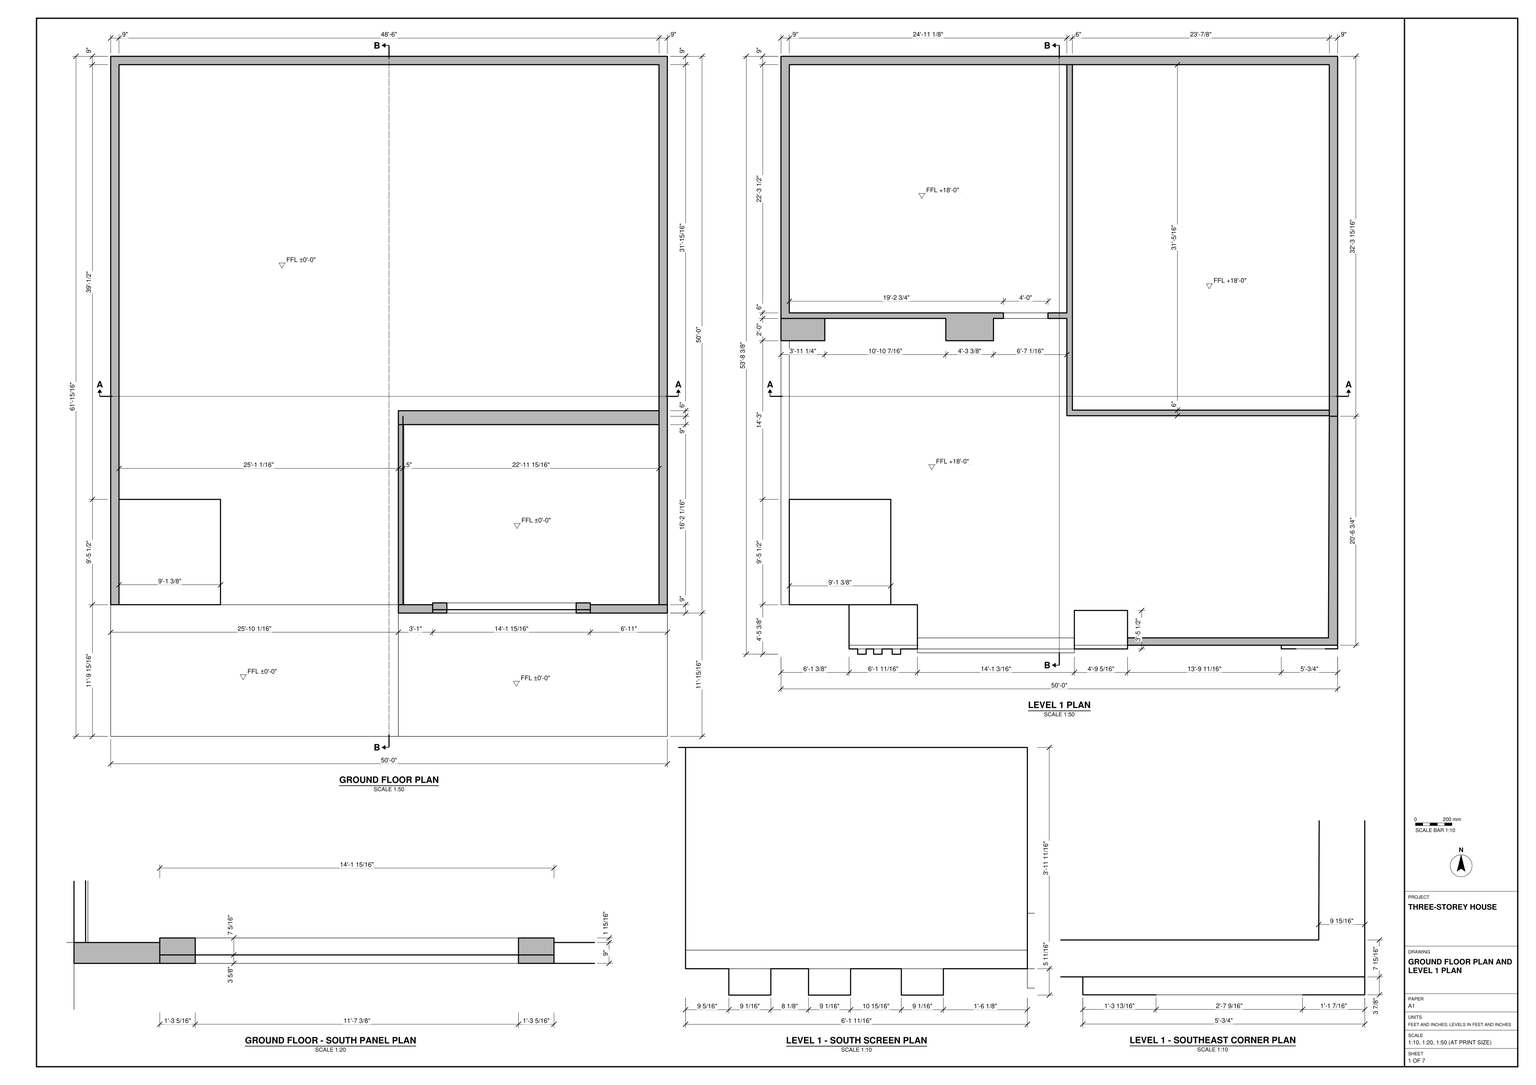
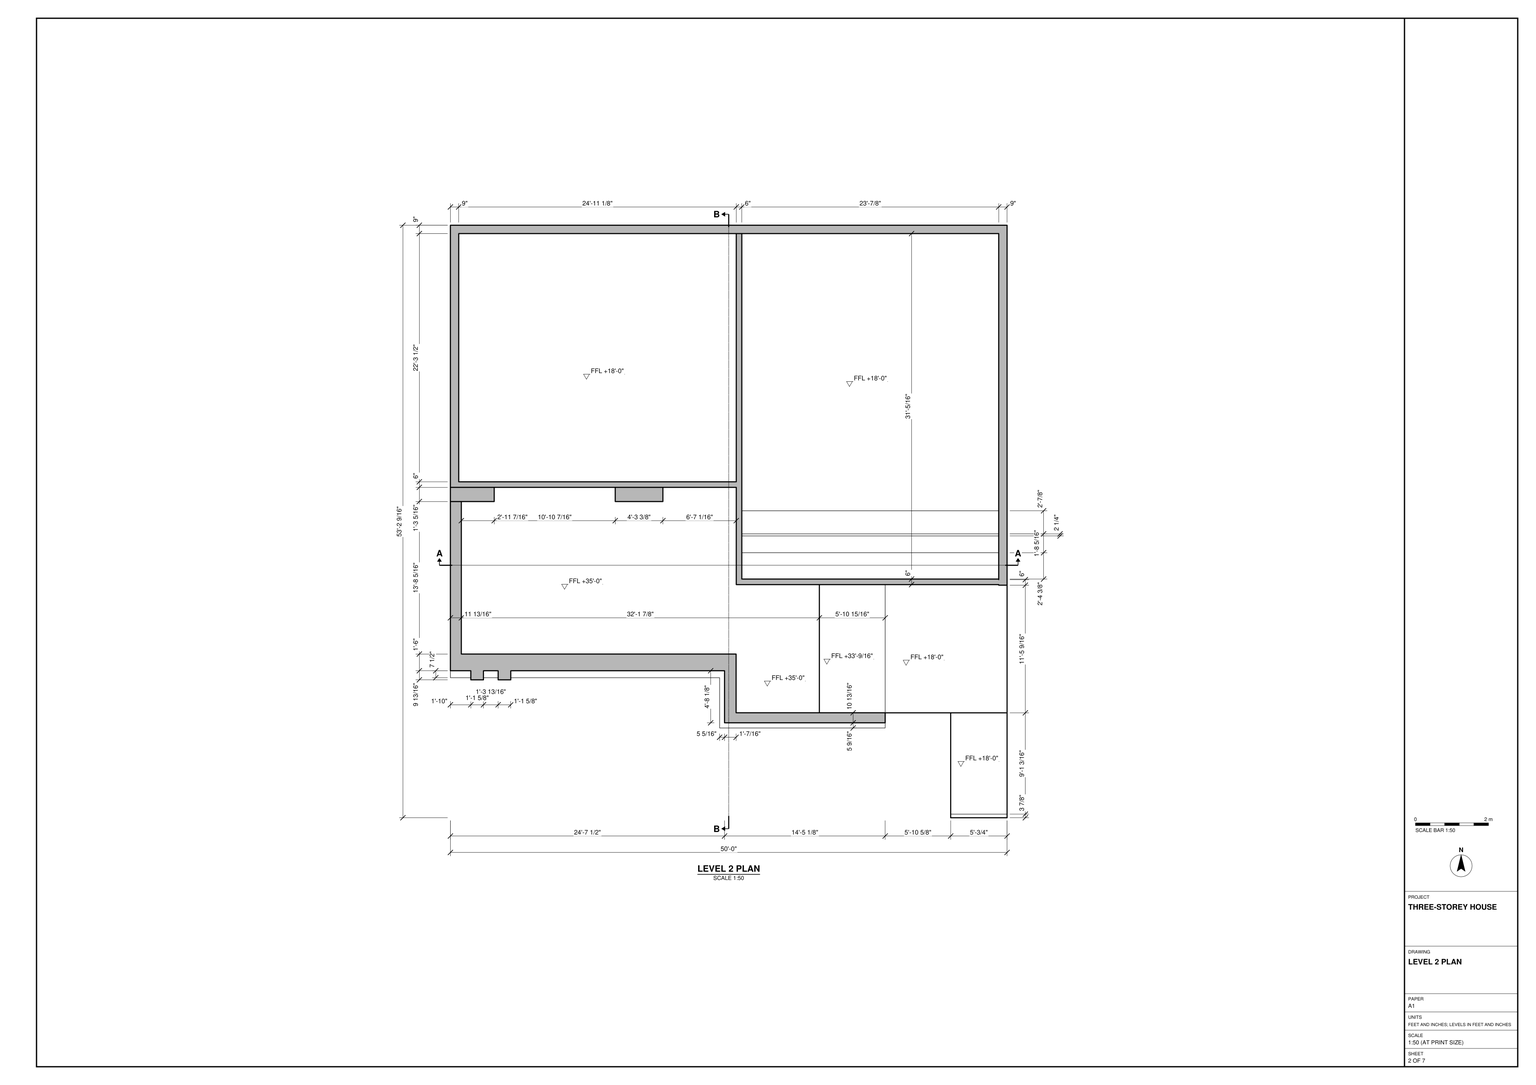
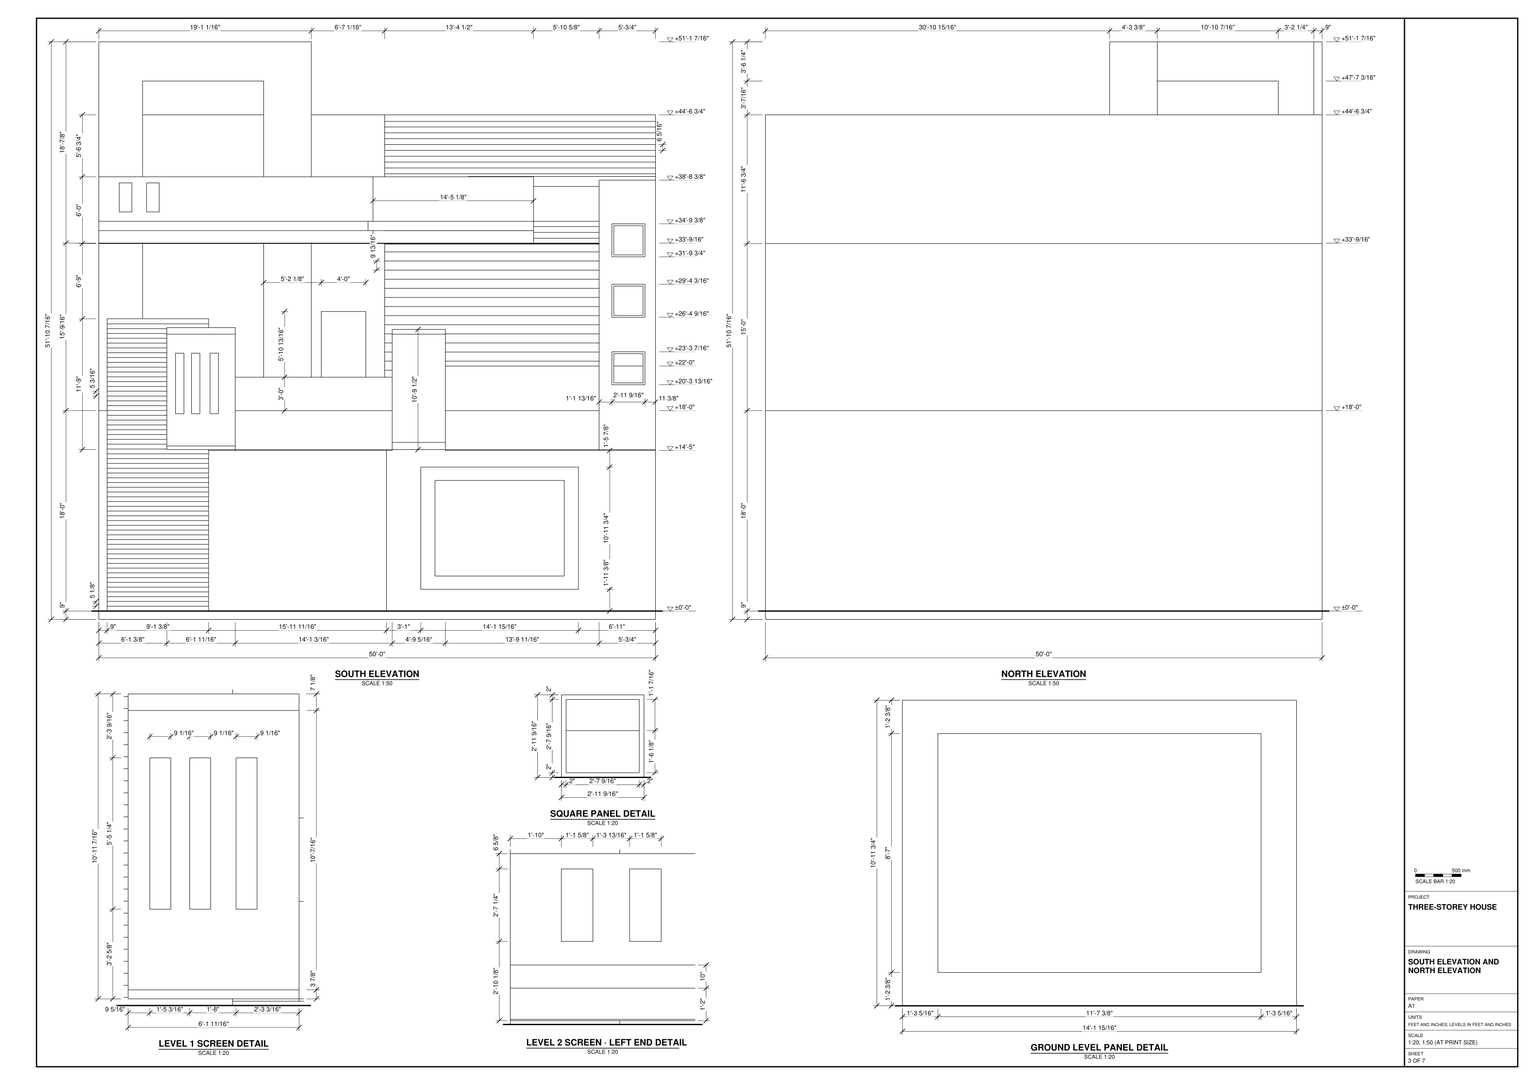
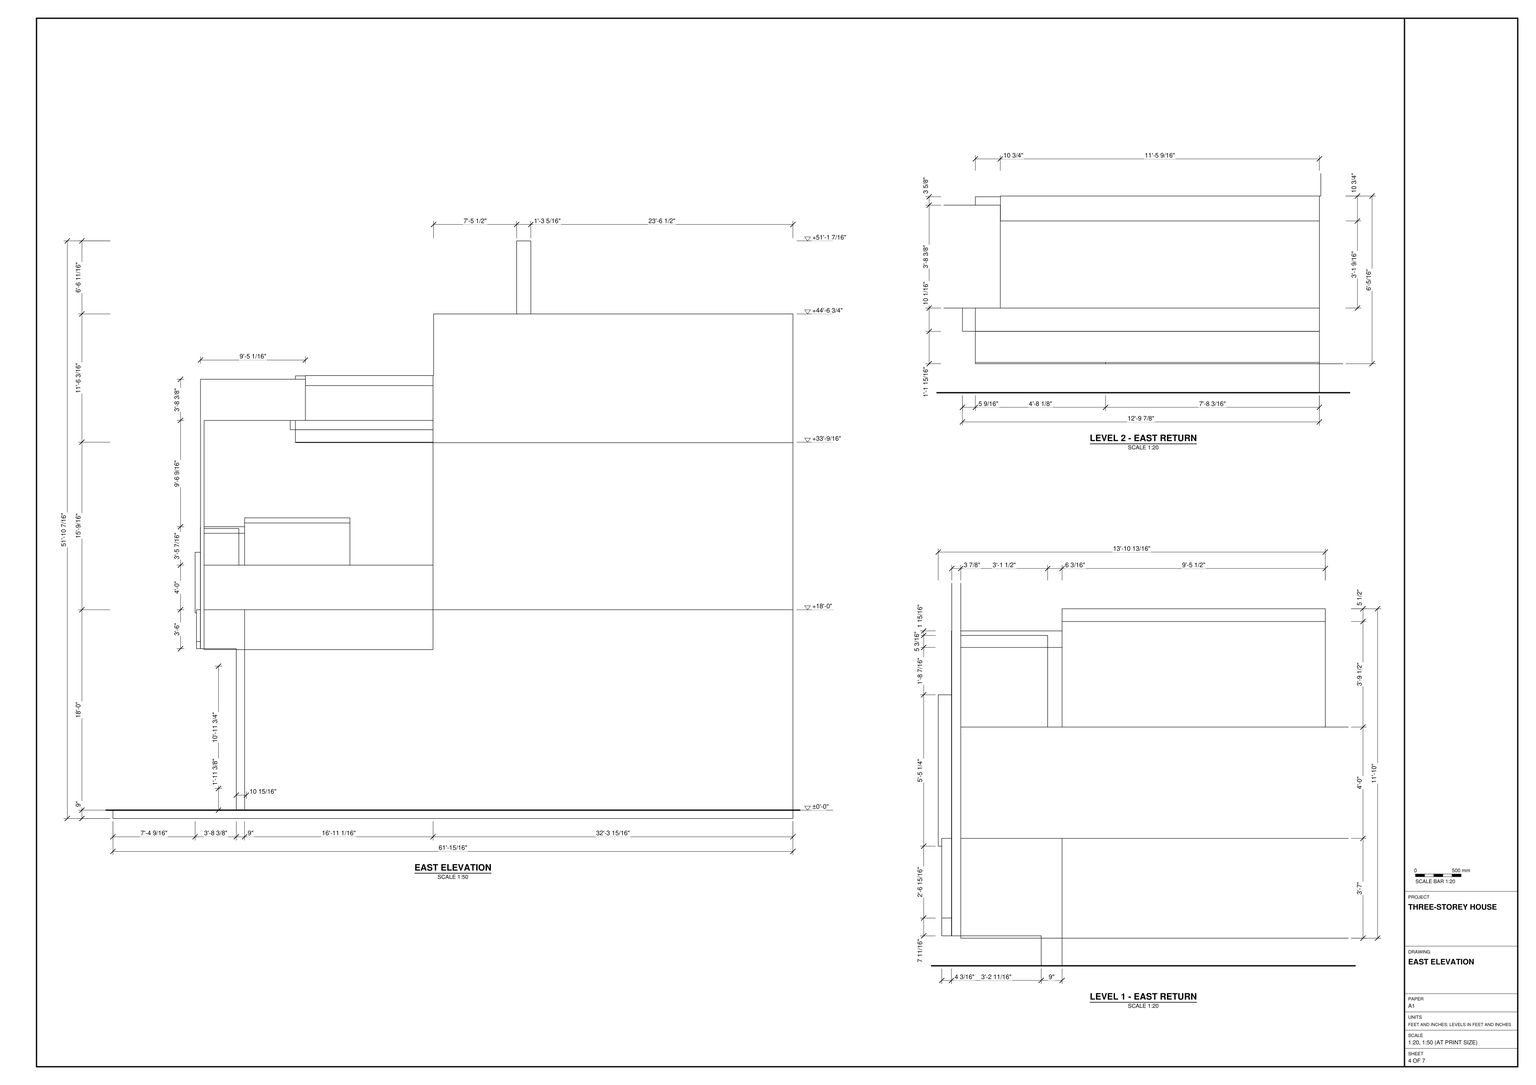
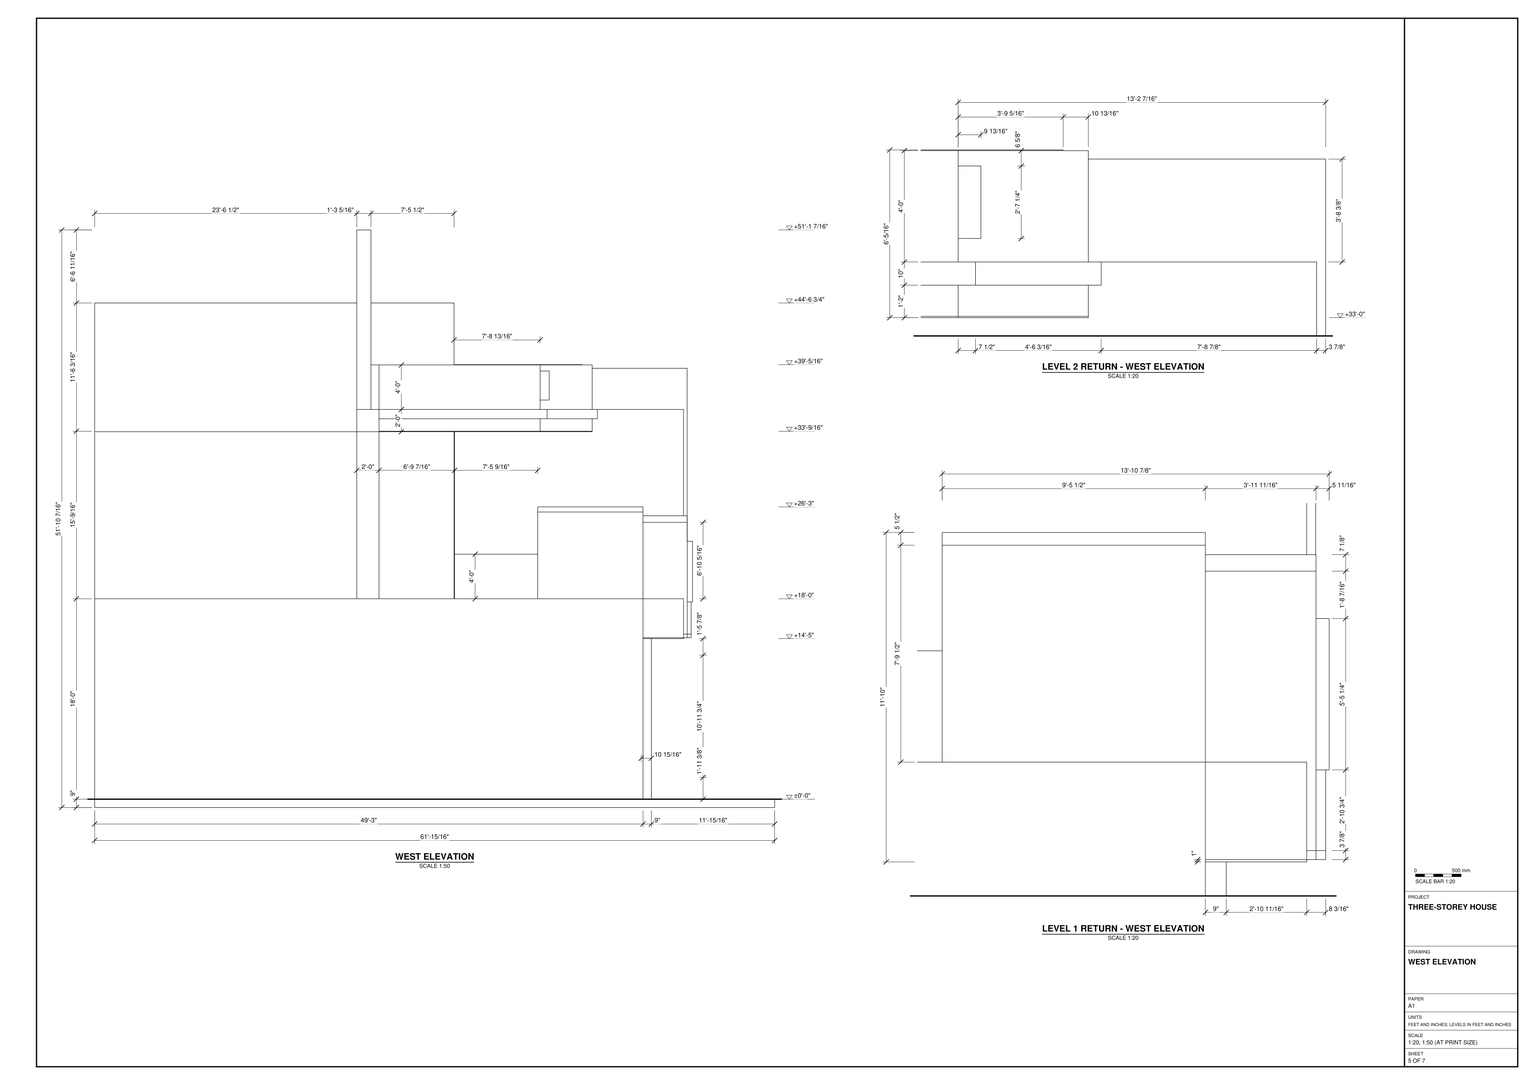
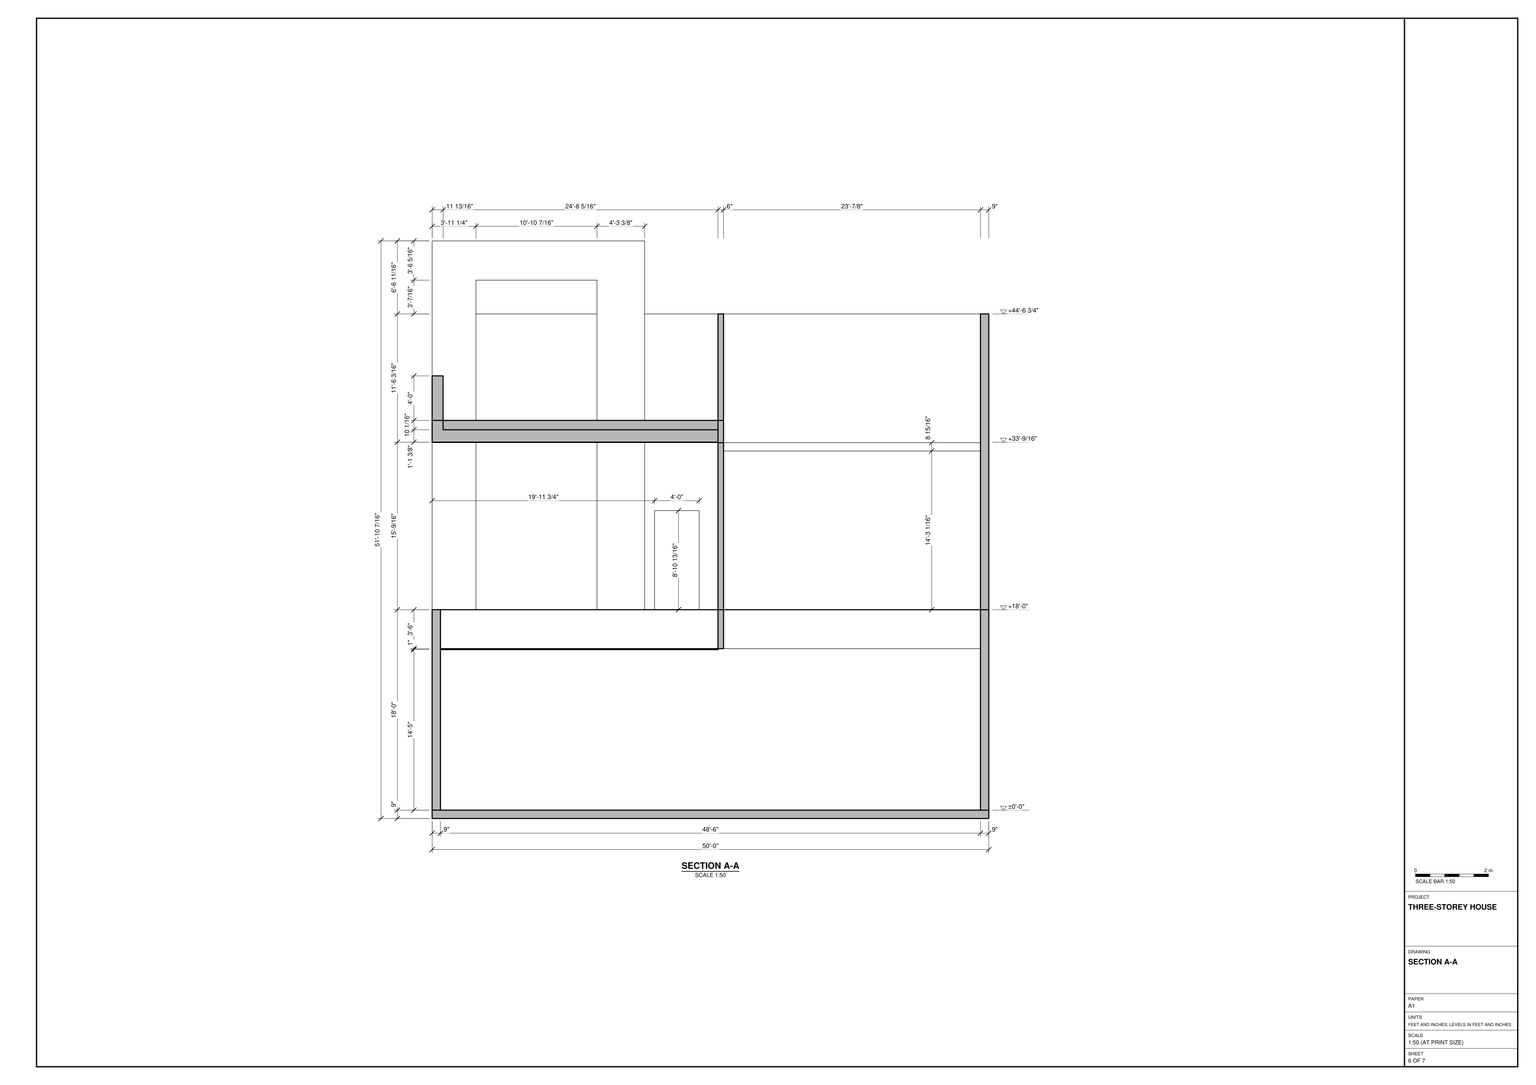
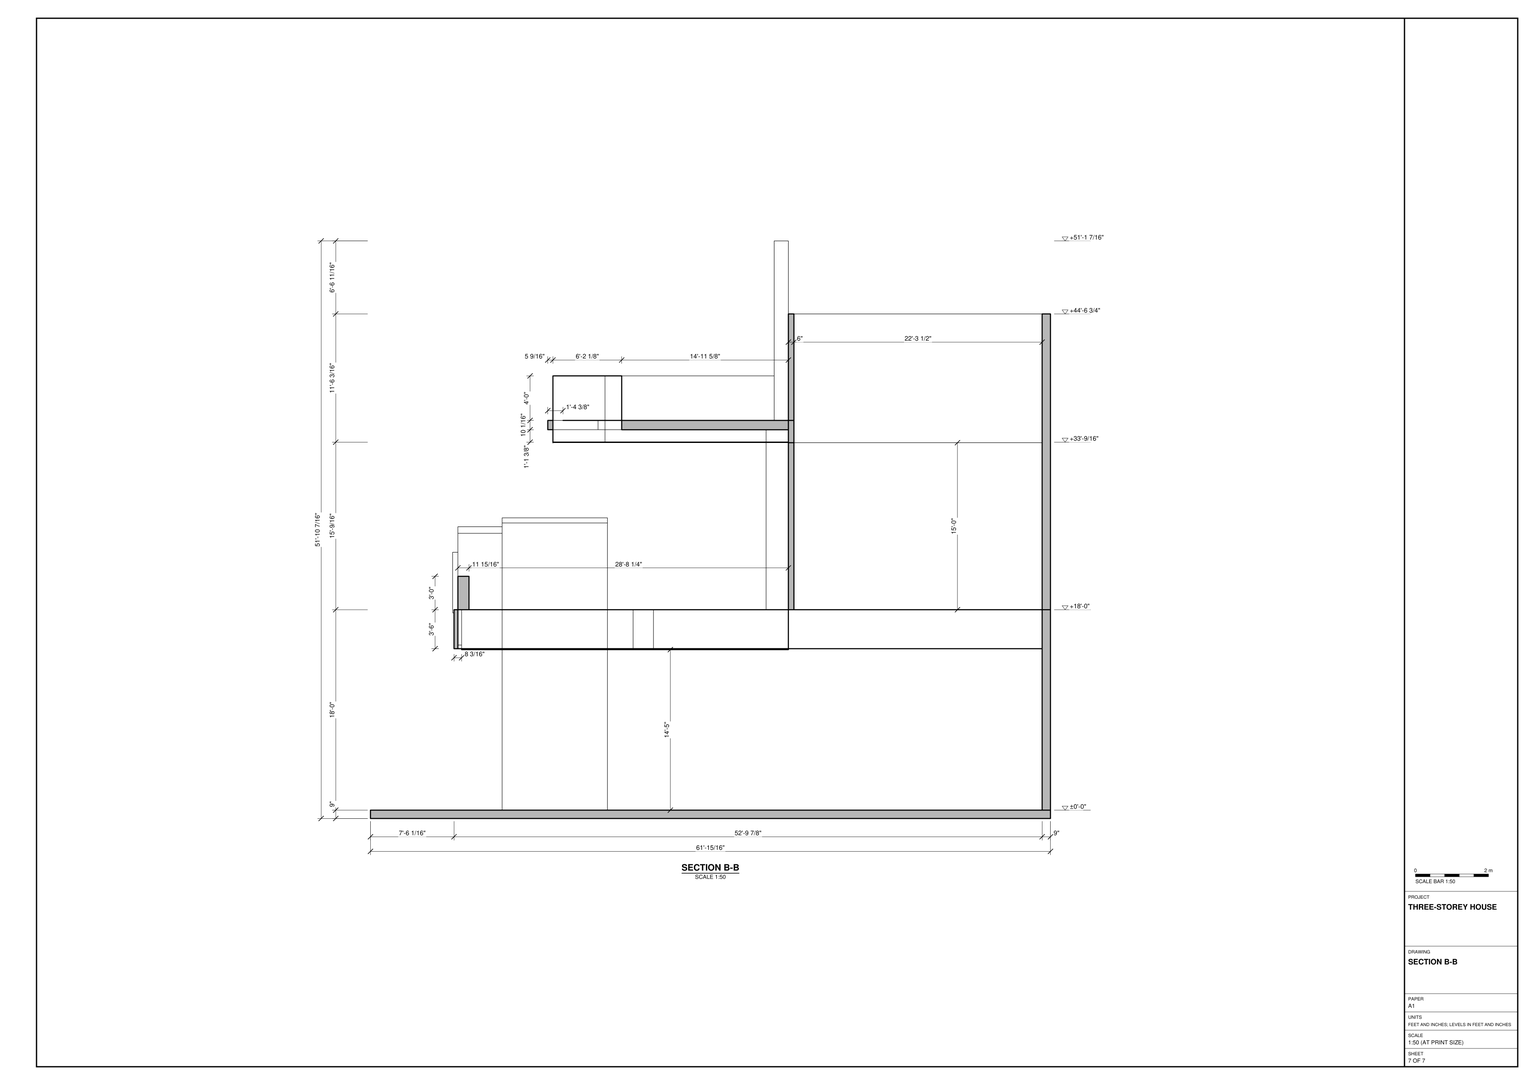
Build the three-storey house in SketchUp from task_files/diagram_01.pdf. Work in feet and inches. The overall extents are 50'-0" east to west, 61'-15/16" north to south and 51'-10 7/16" vertically. Set the finished floor levels to ±0'-0", +18'-0" and +33'-9/16" relative to the ground floor.

Begin with the rectangular base. Lay out the ground-floor walls so that the enclosed southeast bay sits beside the open area to its west. At the next level, follow the two rear enclosures: they share a dividing wall, but the eastern enclosure extends farther south. Use the wall thicknesses shown in plan. Match the slab edges, openings, setbacks and roof profile to the plans and elevations rather than repeating one footprint at every storey.

Use the enlarged details to model the depth of the south façade. Include the large framed ground-floor panel, the horizontally banded surfaces, the projecting screen with three narrow vertical strips and the stacked square panels at the southeast corner. Keep the north face plain as drawn.

Make walls, slabs, roof elements and any furniture or joinery shown separate groups or components. Use components for repeated parts. Any decor or loose items shown may be suitable library components. Save one SketchUp model as output_files/three_storey_house_with_stepped_south_facade.skp.

# SketchUp Ruby script. Lengths in inches.
U = 1.inch
M = Sketchup.active_model
def pt(a) = Geom::Point3d.new(a.map { |v| v * U })
def face(e, loops, mat)
  f = e.add_face(loops[0].map { |a| pt(a) })
  loops[1..].each { |l| e.add_face(l.map { |a| pt(a) }).erase! }
  f.material = f.back_material = mat if mat
  f
end
# faces: each face lists its corners as indices into pts; further lists are holes
def faces(e, pts, list, mat = nil) = list.each { |f| face(e, (f[0].is_a?(Array) ? f : [f]).map { |l| l.map { |i| pts[i] } }, mat) }
# xy, xz, yz: faces in a plane at the given z, y or x. An outline is a flat list of corners, or four numbers for a rectangle; further outlines are holes
def ring(l) = l.size == 4 ? [[l[0], l[1]], [l[2], l[1]], [l[2], l[3]], [l[0], l[3]]] : l.each_slice(2).to_a
def flat(e, list, mat, &to3) = list.each { |f| face(e, (f[0].is_a?(Array) ? f : [f]).map { |l| ring(l).map { |u, v| to3.(u, v) } }, mat) }
def xy(e, z, list, mat = nil) = flat(e, list, mat) { |x, y| [x, y, z] }
def xz(e, y, list, mat = nil) = flat(e, list, mat) { |x, z| [x, y, z] }
def yz(e, x, list, mat = nil) = flat(e, list, mat) { |y, z| [x, y, z] }
def lines(e, pts, list) = list.each { |a, b| e.add_line(pt(pts[a]), pt(pts[b])) }
# prism: a flat outline (further loops are holes) pulled along v
def prism(e, loops, v, mat = nil)
  f = face(e, loops, mat); d = Geom::Vector3d.new(v.map { |x| x * U })
  f.pushpull(f.normal.samedirection?(d) ? d.length : -d.length)
end
def box(e, o, s, mat = nil) = prism(e, [[o, [o[0] + s[0], o[1], o[2]], [o[0] + s[0], o[1] + s[1], o[2]], [o[0], o[1] + s[1], o[2]]]], [0, 0, s[2]], mat)
def at(x, y, z, deg = 0) = Geom::Transformation.translation(pt([x, y, z])) * Geom::Transformation.rotation(ORIGIN, Z_AXIS, deg.degrees)
def axes(o, x, y, z) = Geom::Transformation.new([*x, 0, *y, 0, *z, 0, *pt(o).to_a, 1])
def part(name) = M.definitions.add(name)
# library, detail: a bought-in or finely detailed component or shape, given as its bounding box
def library(name, o, s) = part(name).tap { |d| box(d.entities, o, s) }
def detail(e, o, s) = box(e.add_group.entities, o, s)
def put(e, d, t, mat = nil) = e.add_instance(d, t).tap { |i| i.material = mat if mat }
def group(e, t, mat = nil) = e.add_group.tap { |g| g.transformation = t; g.material = mat if mat }.entities
root = M.entities
M.materials.add("[Color D08]").color = [102, 76, 0]
M.materials.add("[Color M00]").color = [255, 255, 255]
M.materials.add("[Color M03]").color = [170, 170, 170]
M.materials.add("[Color M06]").color = [86, 86, 86]
M.materials.add("[Translucent Glass Blue]").color = [100, 149, 237]
M.materials["[Translucent Glass Blue]"].alpha = 0.5
M.materials.add("[Wood Floor Parquet]").color = [145, 89, 39]
xy(root,0,[[0,0,600,732.9375]])
xy(root,9,[[0,0,310.0625,141.9375],[310.0625,0,600,132.9375],[310.0625,132.9375,600,141.9375],[0,141.9375,0,732.9375,600,732.9375,600,141.9375,591,141.9375,591,723.9375,9,723.9375,9,141.9375],[118.375,141.9375,310.0625,141.9375,310.0625,351,591,351,591,723.9375,9,723.9375,9,255.41,118.375,255.41],
  [310.0625,141.9375,315.0625,336],[315.0625,141.9375,316.0625,336],[316.0625,141.9375,591,336],[310.0625,336,315.0625,340.1875],[315.0625,336,316.0625,340.1875],
  [315.0625,336,316.0625,345],[316.0625,336,591,340.1875],[310.0625,340.1875,315.0625,345],[315.0625,340.1875,316.0625,345],[316.0625,340.1875,591,345],
  [310.0625,345,591,351]])
xy(root,32.36,[[347.05,132.9375,516.98,141.9375]])
xy(root,164.11,[[347.05,132.9375,516.98,141.9375]])
xy(root,182,[[147.0625,98.25,147.0625,141.9375,118.375,141.9375,118.375,255.41,9,255.41,9,450.4375,308.125,450.4375,308.125,345.625,591,345.625,591,345,600,345,600,98.25,373.53,98.25,373.53,135.73,316.23,135.73,316.23,98.25]])
xy(root,183,[[147.0625,94.25,316.23,98.25],[539.23,94.375,600,98.25],[73.375,98.25,73.375,141.9375,118.375,141.9375,118.375,255.41,9,255.41,9,723.9375,314.125,723.9375,314.125,351.625,591,351.625,591,351,310.0625,351,310.0625,132.9375,600,132.9375,600,98.25],[310.0625,141.9375,315.0625,336],[310.0625,336,315.0625,340.1875],
  [315.0625,336,591,340.1875],[310.0625,340.1875,315.0625,345],[315.0625,340.1875,591,340.1875,591,351,310.0625,351,310.0625,345,315.0625,345]])
xy(root,183,[[147.0625,90.0625,316.23,94.25]],"[Color M03]")
xy(root,186.875,[[73.375,94.25,147.0625,98.25]])
xy(root,189,[[310.0625,132.9375,316.0625,141.9375]])
xy(root,190.6875,[[316.23,94.25,373.53,98.25]])
xy(root,221.65,[[82.71,88.5625,91.77,94.25],[99.9,88.5625,108.96,94.25],[119.9,88.5625,128.96,94.25]],"[Color M00]")
xy(root,225,[[147.0625,94.25,316.23,106.2],[73.375,98.25,147.0625,141.9375],[316.23,98.25,373.53,135.73],[373.53,98.25,373.53,106.2,590.08,106.2,591,345,600,345,600,98.25],[147.0625,106.2,316.23,106.2,316.23,135.73,373.53,135.73,373.53,106.2,590.08,106.2,591,345,591,345.625,308.125,345.625,308.125,450.4375,229.06,450.4375,229.06,426.4375,177.67,426.4375,177.67,450.4375,47.22,450.4375,47.22,426.4375,9,426.4375,9,255.41,118.375,255.41,118.375,141.9375,147.0625,141.9375],
  [0,141.9375,9,426.4375],[591,345,591,723.9375,9,723.9375,9,450.4375,0,450.4375,0,732.9375,600,732.9375,600,345],[308.125,345.625,308.125,450.4375,287.77,450.4375,287.77,456.4375,308.125,456.4375,308.125,723.9375,314.125,723.9375,314.125,351.625,591,351.625,591,345.625],[314.125,351.625,591,723.9375],[0,426.4375,9,450.4375],
  [9,426.4375,47.22,450.4375],[177.67,426.4375,229.06,450.4375],[9,450.4375,239.77,456.4375],[239.77,450.4375,287.77,456.4375],[9,456.4375,308.125,723.9375]])
xy(root,225,[[147.0625,90.0625,316.23,94.25]],"[Color M03]")
xy(root,261,[[147.0625,94.25,316.23,106.2]])
xy(root,273,[[373.53,98.25,600,98.25,600,345,591,345,590.08,106.2,373.53,106.2]])
xy(root,286.9,[[82.71,88.5625,91.77,94.25],[99.9,88.5625,108.96,94.25],[119.9,88.5625,128.96,94.25]],"[Color M00]")
xy(root,307.3125,[[73.375,94.25,147.0625,141.9375],[316.23,94.25,373.53,135.73]])
xy(root,312.5,[[316.23,94.25,373.53,135.73]])
xy(root,314.4375,[[73.375,94.25,147.0625,141.9375]])
xy(root,318.5,[[9,141.9375,118.375,255.41]])
xy(root,324,[[9,141.9375,118.375,255.41]])
xy(root,331.8125,[[239.77,450.4375,287.77,456.4375]])
xy(root,405,[[308.125,345.625,308.125,450.4375,9,450.4375,9,456.4375,308.125,456.4375,308.125,723.9375,314.125,723.9375,314.125,351.625,591,351.625,591,345.625],[0,426.4375,9,450.4375],[9,426.4375,47.22,450.4375],[177.67,426.4375,229.06,450.4375]])
xy(root,405.5625,[[295.5,196.6875,468.62,196.6875,468.62,345,591,345,591,345.625,308.125,345.625,308.125,450.4375,229.06,450.4375,229.06,426.4375,177.67,426.4375,177.67,450.4375,47.22,450.4375,47.22,426.4375,0,426.4375,0,252.8125,295.5,252.8125]],"[Color M00]")
xy(root,418.9375,[[307.9375,196.6875,307.9375,270.8,11.8,270.8,11.8,435.14,47.22,435.14,47.22,450.4375,177.67,450.4375,177.67,435.14,229.06,435.14,229.06,450.4375,308.125,450.4375,308.125,345.625,468.62,345.625,468.62,196.6875]])
xy(root,419,[[290.1875,191.125,290.1875,245.3125,0,245.3125,0,252.8125,295.5,252.8125,295.5,196.6875,468.62,196.6875,468.62,191.125]])
xy(root,429,[[539.23,98.25,600,207.45],[290.1875,191.125,468.62,191.125,468.62,196.6875,295.5,196.6875,295.5,252.8125,0,252.8125,0,245.3125,290.1875,245.3125],[307.9375,196.6875,468.62,207.51],[468.62,207.45,468.62,345.625,591,345.625,591,345,600,345,600,207.45],[295.5,207.51,295.5,252.8125,0,252.8125,0,435.14,11.8,435.14,11.8,270.8,307.9375,270.8,307.9375,207.51],
  [307.9375,207.51,397.69,207.51,397.69,345.625,308.125,345.625,308.125,450.4375,229.06,450.4375,229.06,435.14,177.67,435.14,177.67,450.4375,47.22,450.4375,47.22,435.14,11.8,435.14,11.8,270.8,307.9375,270.8],[397.69,207.51,468.62,345.625],[308.125,345.625,308.125,450.4375,9,450.4375,9,456.4375,308.125,456.4375,308.125,723.9375,314.125,723.9375,314.125,351.625,591,351.625,591,345.625],[0,435.14,47.22,450.4375],[177.67,435.14,229.06,450.4375]])
xy(root,439.15,[[22.03,243,35.65,252.8125],[51.47,243,65.09,252.8125]])
xy(root,466.5625,[[468.62,207.45,600,207.51],[397.69,207.51,397.69,345.625,591,345.625,591,345,600,345,600,207.51]])
xy(root,470.4,[[22.03,243,35.65,252.8125],[51.47,243,65.09,252.8125]])
xy(root,473.375,[[539.23,94.375,600,207.45]],"[Wood Floor Parquet]")
xy(root,477,[[295.5,196.6875,468.62,196.6875,468.62,207.51,307.9375,207.51,307.9375,270.8,11.8,270.8,11.8,435.14,0,435.14,0,252.8125,295.5,252.8125]])
xy(root,477.3125,[[397.69,207.51,600,207.51,600,345,591,345,591,345.625,397.69,345.625],[591,345,600,345.625]])
xy(root,543.75,[[591,345.625,600,345.625,600,732.9375,0,732.9375,0,450.4375,9,450.4375,9,723.9375,591,723.9375],[308.125,345.625,591,345.625,591,351.625,314.125,351.625,314.125,723.9375,308.125,723.9375,308.125,456.4375,9,456.4375,9,450.4375,308.125,450.4375]])
xy(root,580.16,[[47.22,435.14,177.67,450.4375]],"[Wood Floor Parquet]")
xy(root,622.4375,[[0,435.14,229.06,450.4375]],"[Wood Floor Parquet]")
xz(root,0,[[0,0,600,9]])
xz(root,88.5625,[[82.71,221.65,91.77,286.9],[99.9,221.65,108.96,286.9],[119.9,221.65,128.96,286.9]],"[Color M00]")
xz(root,90.0625,[[147.0625,183,316.23,225]],"[Color M00]")
xz(root,94.25,[[73.375,307.3125,147.0625,314.4375],[316.23,307.3125,373.53,312.5]])
xz(root,94.25,[[147.0625,183,316.23,225],[147.0625,225,316.23,261]],"[Color M03]")
xz(root,94.25,[[[73.375,186.875,147.0625,307.3125],[82.71,221.65,91.77,286.9],[99.9,221.65,108.96,286.9],[119.9,221.65,128.96,286.9]],[316.23,190.6875,373.53,307.3125]],"[Wood Floor Parquet]")
xz(root,94.375,[[[553.02,252.84,588.6,288.42],[555.03,254.85,586.59,286.41]],[[553.02,325.59,588.6,361.17],[555.03,327.6,586.59,359.16]],[[553.02,390.78,588.6,426.36],[555.03,392.79,586.59,424.35]]],"[Color M00]")
xz(root,94.375,[[[539.23,183,600,473.375],[553.02,390.78,588.6,426.36],[553.02,325.59,588.6,361.17],[553.02,252.84,588.6,288.42]],[555.03,392.79,586.59,424.35]],"[Wood Floor Parquet]")
xz(root,98.25,[[147.0625,182,316.23,183],[373.53,182,539.23,183],[539.23,182,600,183],[73.375,183,147.0625,186.875],[316.23,183,373.53,190.6875],
  [373.53,183,539.23,225],[539.23,183,600,225],[73.375,186.875,147.0625,225],[316.23,190.6875,373.53,225],[539.23,225,600,273],
  [539.23,273,600,429]])
xz(root,98.25,[[373.53,225,539.23,273]],"[Color M03]")
xz(root,106.2,[[147.0625,225,316.23,261],[373.53,225,590.08,273]])
xz(root,132.9375,[[[310.0625,9,600,183],[347.05,32.36,516.98,164.11]],[310.0625,183,316.0625,189]])
xz(root,135.73,[[316.23,182,373.53,225],[316.23,307.3125,373.53,312.5]])
xz(root,135.73,[[316.23,225,373.53,307.3125]],"[Wood Floor Parquet]")
xz(root,141.9375,[[0,9,9,225],[9,9,118.375,9.125],[310.0625,9,315.0625,183],[315.0625,9,316.0625,183],[[316.0625,9,591,183],[347.05,32.36,516.98,164.11]],
  [591,9,600,189],[118.375,182,147.0625,225],[73.375,183,118.375,183.625],[310.0625,183,316.0625,189],[316.0625,183,591,189],
  [73.375,183.625,118.375,188.8125],[73.375,188.8125,118.375,194],[73.375,194,118.375,199.1875],[73.375,199.1875,118.375,204.375],[73.375,204.375,118.375,209.5625],
  [73.375,209.5625,118.375,214.75],[73.375,214.75,118.375,219.9375],[73.375,219.9375,118.375,225],[73.375,225,118.375,225.125],[73.375,225.125,118.375,230.3125],
  [73.375,230.3125,118.375,235.5],[73.375,235.5,118.375,240.6875],[73.375,240.6875,118.375,245.875],[73.375,245.875,118.375,251.0625],[73.375,251.0625,118.375,256.25],
  [73.375,256.25,118.375,261.4375],[73.375,261.4375,118.375,266.625],[73.375,266.625,118.375,271.8125],[73.375,271.8125,118.375,277],[73.375,277,118.375,282.1875],
  [73.375,282.1875,118.375,287.375],[73.375,287.375,118.375,292.5625],[73.375,292.5625,118.375,297.75],[73.375,297.75,118.375,302.9375],[73.375,302.9375,118.375,307.3125],
  [73.375,307.3125,118.375,308.125],[118.375,307.3125,147.0625,314.4375],[73.375,308.125,118.375,313.3125],[73.375,313.3125,118.375,314.4375],[9,318.5,118.375,324]])
xz(root,141.9375,[[9,9.125,118.375,14.25],[9,14.25,118.375,19.375],[9,19.375,118.375,24.5],[9,24.5,118.375,29.625],[9,29.625,118.375,34.75],
  [9,34.75,118.375,39.875],[9,39.875,118.375,45],[9,45,118.375,50.125],[9,50.125,118.375,55.25],[9,55.25,118.375,60.375],
  [9,60.375,118.375,65.5],[9,65.5,118.375,70.625],[9,70.625,118.375,75.75],[9,75.75,118.375,80.875],[9,80.875,118.375,86],
  [9,86,118.375,91.125],[9,91.125,118.375,96.25],[9,96.25,118.375,101.375],[9,101.375,118.375,106.5],[9,106.5,118.375,111.625],
  [9,111.625,118.375,116.75],[9,116.75,118.375,121.875],[9,121.875,118.375,127],[9,127,118.375,132.125],[9,132.125,118.375,137.25],
  [9,137.25,118.375,142.375],[9,142.375,118.375,147.5],[9,147.5,118.375,152.625],[9,152.625,118.375,157.75],[9,157.75,118.375,162.875],
  [9,162.875,118.375,168.0625],[9,168.0625,118.375,173.25],[9,173.25,118.375,178.4375],[9,178.4375,118.375,178.4375,118.375,183,73.375,183,73.375,183.625,9,183.625],[9,183.625,73.375,188.8125],
  [9,188.8125,73.375,194],[9,194,73.375,199.1875],[9,199.1875,73.375,204.375],[9,204.375,73.375,209.5625],[9,209.5625,73.375,214.75],
  [9,214.75,73.375,219.9375],[9,219.9375,73.375,225.125],[9,225.125,73.375,230.3125],[9,230.3125,73.375,235.5],[9,235.5,73.375,240.6875],
  [9,240.6875,73.375,245.875],[9,245.875,73.375,251.0625],[9,251.0625,73.375,256.25],[9,256.25,73.375,261.4375],[9,261.4375,73.375,266.625],
  [9,266.625,73.375,271.8125],[9,271.8125,73.375,277],[9,277,73.375,282.1875],[9,282.1875,73.375,287.375],[9,287.375,73.375,292.5625],
  [9,292.5625,73.375,297.75],[9,297.75,73.375,302.9375],[9,302.9375,73.375,308.125],[9,308.125,73.375,313.3125],[9,313.3125,73.375,313.3125,73.375,314.4375,118.375,314.4375,118.375,318.5,9,318.5]],"[Color M06]")
xz(root,141.9375,[[118.375,225,147.0625,307.3125]],"[Wood Floor Parquet]")
xz(root,191.125,[[290.1875,419,468.62,429]])
xz(root,196.6875,[[295.5,405,468.62,405.5625],[295.5,405.5625,468.62,405.5625,468.62,418.9375,307.9375,418.9375,307.9375,419,295.5,419],[307.9375,418.9375,468.62,419],[295.5,419,307.9375,429],[307.9375,419,468.62,429]])
xz(root,196.6875,[[295.5,429,468.62,477]],"[Color M03]")
xz(root,207.45,[[468.62,429,539.23,466.5625],[539.23,429,600,466.5625],[539.23,466.5625,600,473.375]])
xz(root,207.51,[[307.9375,429,397.69,477],[397.69,429,468.62,466.5625],[397.69,466.5625,468.62,477],[468.62,466.5625,600,466.5625,600,477.3125,397.69,477.3125,397.69,477,468.62,477]])
xz(root,243,[[22.03,439.15,35.65,470.4],[51.47,439.15,65.09,470.4]])
xz(root,245.3125,[[0,419,290.1875,429]])
xz(root,252.8125,[[0,405,295.5,405.5625],[0,405.5625,295.5,419]])
xz(root,252.8125,[[[0,429,295.5,477],[22.03,439.15,35.65,470.4],[51.47,439.15,65.09,470.4]]],"[Color M03]")
xz(root,255.41,[[9,9,118.375,182],[9,182,118.375,183],[9,183,118.375,225],[9,318.5,118.375,324]])
xz(root,255.41,[[9,225,118.375,318.5]],"[Color M06]")
xz(root,270.8,[[11.8,418.9375,307.9375,429],[11.8,429,307.9375,477]])
xz(root,336,[[310.0625,9,591,183]])
xz(root,345,[[591,182,600,225],[591,225,600,273],[591,273,600,405],[591,405,600,429],[591,429,600,466.5625],
  [591,466.5625,600,477.3125]])
xz(root,345.625,[[308.125,182,591,199.79],[308.125,199.79,591,209.6],[308.125,209.6,591,219.41],[308.125,219.41,591,225],[308.125,405,591,405.5625],
  [308.125,418.9375,468.62,419],[308.125,419,468.62,423.37],[308.125,423.37,468.62,429],[308.125,429,397.69,429.68],[397.69,429,591,429.68],
  [397.69,429.68,591,435.99],[397.69,435.99,591,442.31],[397.69,442.31,591,448.62],[397.69,448.62,591,454.93],[397.69,454.93,591,461.24],
  [397.69,461.24,591,466.5625],[397.69,466.5625,591,467.56],[397.69,467.56,591,473.87],[397.69,473.87,591,477.3125]])
xz(root,345.625,[[308.125,404.43,591,405]],"[Color M00]")
xz(root,345.625,[[308.125,225,591,229.22],[308.125,229.22,591,239.04],[308.125,239.04,591,248.85],[308.125,248.85,591,258.66],[308.125,258.66,591,268.47],
  [308.125,268.47,591,278.29],[308.125,278.29,591,288.1],[308.125,288.1,591,297.91],[308.125,297.91,591,307.72],[308.125,307.72,591,317.54],
  [308.125,317.54,591,327.35],[308.125,327.35,591,337.16],[308.125,337.16,591,346.97],[308.125,346.97,591,356.79],[308.125,356.79,591,366.6],
  [308.125,366.6,591,376.41],[308.125,376.41,591,386.22],[308.125,386.22,591,396.04],[308.125,396.04,591,404.43],[308.125,405.5625,591,410.74],
  [308.125,410.74,591,417.06],[308.125,417.06,308.125,418.9375,468.62,418.9375,468.62,423.37,591,423.37,591,417.06],[468.62,423.37,591,429],[308.125,429.68,397.69,435.99],[308.125,435.99,397.69,442.31],
  [308.125,442.31,397.69,448.62],[308.125,448.62,397.69,454.93],[308.125,454.93,397.69,461.24],[308.125,461.24,397.69,467.56],[308.125,467.56,397.69,473.87],
  [308.125,473.87,397.69,473.87,397.69,477.3125,600,477.3125,600,480.18,308.125,480.18],[308.125,480.18,600,486.49],[308.125,486.49,600,492.81],[308.125,492.81,600,499.12],[308.125,499.12,600,505.43],
  [308.125,505.43,600,511.74],[308.125,511.74,600,518.06],[308.125,518.06,600,524.37],[308.125,524.37,600,530.68],[308.125,530.68,600,536.68],
  [308.125,536.68,600,543.75]],"[Color M06]")
xz(root,351,[[310.0625,9,591,183]])
xz(root,351.625,[[314.125,183,591,225],[314.125,225,591,405],[314.125,405,591,429],[314.125,429,591,543.75]])
xz(root,426.4375,[[0,405,9,405.5625],[9,405,47.22,405.5625],[177.67,405,229.06,405.5625],[0,405.5625,9,419],[9,405.5625,47.22,419],
  [177.67,405.5625,229.06,419]])
xz(root,426.4375,[[0,225,47.22,405],[177.67,225,229.06,405]],"[Wood Floor Parquet]")
xz(root,435.14,[[11.8,418.9375,47.22,429],[177.67,418.9375,229.06,429],[0,429,11.8,477]])
xz(root,435.14,[[11.8,429,47.22,429,47.22,580.16,177.67,580.16,177.67,429,229.06,429,229.06,622.4375,0,622.4375,0,477,11.8,477]],"[Wood Floor Parquet]")
xz(root,450.4375,[[9,182,308.125,225],[0,225,47.22,405],[47.22,225,177.67,405],[229.06,225,239.77,225,239.77,331.8125,287.77,331.8125,287.77,225,308.125,225,308.125,405,229.06,405],[0,405,47.22,429],
  [47.22,405,177.67,405.5625],[177.67,405,229.06,429],[229.06,405,308.125,405.5625],[47.22,405.5625,177.67,418.9375],[229.06,405.5625,308.125,418.9375],
  [47.22,418.9375,177.67,419],[229.06,418.9375,308.125,419],[47.22,419,177.67,429],[229.06,419,308.125,429],[0,429,9,543.75],
  [9,429,47.22,543.75],[47.22,429,177.67,543.75],[177.67,429,229.06,543.75],[229.06,429,308.125,543.75]])
xz(root,450.4375,[[0,543.75,9,622.4375],[9,543.75,9,622.4375,177.67,622.4375,177.67,580.16,47.22,580.16,47.22,543.75],[177.67,543.75,229.06,622.4375]],"[Wood Floor Parquet]")
xz(root,456.4375,[[9,225,9,405,308.125,405,308.125,225,287.77,225,287.77,331.8125,239.77,331.8125,239.77,225],[9,405,308.125,429],[9,429,308.125,543.75]])
xz(root,723.9375,[[9,9,591,183],[9,183,314.125,225],[314.125,183,591,225],[9,225,308.125,405],[308.125,225,314.125,405],
  [314.125,225,591,405],[9,405,308.125,543.75],[308.125,405,314.125,429],[314.125,405,591,543.75],[308.125,429,314.125,543.75]])
xz(root,732.9375,[[0,0,600,9],[0,9,600,225],[0,225,600,405],[0,405,600,543.75]])
yz(root,0,[[0,0,732.9375,9],[141.9375,9,732.9375,225],[450.4375,225,732.9375,405],[252.8125,405,426.4375,405.5625],[450.4375,405,732.9375,543.75],
  [252.8125,405.5625,426.4375,419],[245.3125,419,426.4375,429],[426.4375,429,435.14,477]])
yz(root,0,[[252.8125,429,426.4375,477]],"[Color M03]")
yz(root,0,[[426.4375,225,450.4375,405],[426.4375,405,450.4375,429],[435.14,429,450.4375,622.4375]],"[Wood Floor Parquet]")
yz(root,9,[[141.9375,9,255.41,225],[255.41,9,723.9375,9,723.9375,183,450.4375,183,450.4375,182,255.41,182],[255.41,182,283.09,183],[283.09,182,305.03,183],[305.03,182,450.4375,183],
  [255.41,183,283.09,225],[283.09,183,305.03,225],[305.03,183,450.4375,225],[450.4375,183,723.9375,225],[456.4375,225,723.9375,405],
  [141.9375,318.5,255.41,324],[456.4375,405,723.9375,543.75]])
yz(root,9,[[141.9375,225,255.41,318.5]],"[Color M06]")
yz(root,11.8,[[270.8,418.9375,435.14,429],[270.8,429,435.14,477]])
yz(root,22.03,[[243,439.15,252.8125,470.4]])
yz(root,35.65,[[243,439.15,252.8125,470.4]])
yz(root,47.22,[[426.4375,405,450.4375,405.5625],[426.4375,405.5625,426.4375,419,435.14,419,435.14,418.9375,450.4375,418.9375,450.4375,405.5625],[435.14,418.9375,450.4375,419],[435.14,419,450.4375,429]])
yz(root,47.22,[[426.4375,225,450.4375,405],[435.14,429,450.4375,580.16]],"[Wood Floor Parquet]")
yz(root,51.47,[[243,439.15,252.8125,470.4]])
yz(root,65.09,[[243,439.15,252.8125,470.4]])
yz(root,73.375,[[94.25,307.3125,141.9375,314.4375]])
yz(root,73.375,[[98.25,183,141.9375,225],[94.25,186.875,94.25,307.3125,141.9375,307.3125,141.9375,225,98.25,225,98.25,186.875]],"[Wood Floor Parquet]")
yz(root,82.71,[[88.5625,221.65,94.25,286.9]],"[Color M00]")
yz(root,91.77,[[88.5625,221.65,94.25,286.9]],"[Color M00]")
yz(root,99.9,[[88.5625,221.65,94.25,286.9]],"[Color M00]")
yz(root,108.96,[[88.5625,221.65,94.25,286.9]],"[Color M00]")
yz(root,118.375,[[141.9375,9,255.41,182],[141.9375,182,255.41,183],[141.9375,183,255.41,225],[141.9375,318.5,255.41,324]])
yz(root,118.375,[[141.9375,225,255.41,318.5]],"[Color M06]")
yz(root,119.9,[[88.5625,221.65,94.25,286.9]],"[Color M00]")
yz(root,128.96,[[88.5625,221.65,94.25,286.9]],"[Color M00]")
yz(root,147.0625,[[98.25,182,141.9375,225],[94.25,183,98.25,186.875],[94.25,186.875,98.25,225],[94.25,225,98.25,261],[94.25,307.3125,141.9375,314.4375]])
yz(root,147.0625,[[90.0625,183,94.25,186.875],[90.0625,186.875,94.25,225]],"[Color M03]")
yz(root,147.0625,[[106.2,225,141.9375,225,141.9375,307.3125,94.25,307.3125,94.25,261,106.2,261],[98.25,225,106.2,261]],"[Wood Floor Parquet]")
yz(root,177.67,[[426.4375,405,450.4375,405.5625],[426.4375,405.5625,450.4375,405.5625,450.4375,418.9375,435.14,418.9375,435.14,419,426.4375,419],[435.14,418.9375,450.4375,419],[435.14,419,450.4375,429]])
yz(root,177.67,[[426.4375,225,450.4375,405],[435.14,429,450.4375,580.16]],"[Wood Floor Parquet]")
yz(root,229.06,[[426.4375,405,450.4375,405.5625],[426.4375,405.5625,426.4375,419,435.14,419,435.14,418.9375,450.4375,418.9375,450.4375,405.5625],[435.14,418.9375,450.4375,419],[435.14,419,450.4375,429]])
yz(root,229.06,[[426.4375,225,450.4375,405],[435.14,429,450.4375,622.4375]],"[Wood Floor Parquet]")
yz(root,239.77,[[450.4375,225,456.4375,331.8125]])
yz(root,287.77,[[450.4375,225,456.4375,331.8125]])
yz(root,290.1875,[[191.125,419,245.3125,429]])
yz(root,295.5,[[196.6875,405,252.8125,405.5625],[196.6875,405.5625,252.8125,419],[196.6875,419,245.3125,429],[245.3125,419,252.8125,429]])
yz(root,295.5,[[196.6875,429,245.3125,477],[245.3125,429,252.8125,477]],"[Color M03]")
yz(root,307.9375,[[196.6875,418.9375,270.8,429],[207.51,429,270.8,477]])
yz(root,308.125,[[345.625,182,450.4375,225],[345.625,225,450.4375,405],[456.4375,225,723.9375,405],[345.625,405,450.4375,405.5625],[456.4375,405,723.9375,429],
  [345.625,405.5625,450.4375,418.9375],[345.625,418.9375,450.4375,419],[345.625,419,450.4375,429],[345.625,429,450.4375,543.75],[456.4375,429,723.9375,543.75]])
yz(root,310.0625,[[132.9375,9,141.9375,183],[141.9375,9,336,183],[336,9,351,183],[132.9375,183,141.9375,189]])
yz(root,314.125,[[351.625,183,723.9375,225],[351.625,225,723.9375,405],[351.625,405,723.9375,429],[351.625,429,723.9375,543.75]])
yz(root,315.0625,[[141.9375,9,345,183]])
yz(root,316.23,[[98.25,182,135.73,225],[94.25,183,98.25,190.6875],[94.25,190.6875,98.25,225],[94.25,225,98.25,261],[94.25,307.3125,135.73,312.5]])
yz(root,316.23,[[90.0625,183,94.25,190.6875],[90.0625,190.6875,94.25,225]],"[Color M03]")
yz(root,316.23,[[106.2,225,106.2,261,94.25,261,94.25,307.3125,135.73,307.3125,135.73,225],[98.25,225,106.2,261]],"[Wood Floor Parquet]")
yz(root,347.05,[[132.9375,32.36,141.9375,164.11]])
yz(root,373.53,[[98.25,182,135.73,225],[98.25,225,106.2,273],[94.25,307.3125,135.73,312.5]])
yz(root,373.53,[[94.25,190.6875,98.25,190.6875,98.25,273,106.2,273,106.2,225,135.73,225,135.73,307.3125,94.25,307.3125]],"[Wood Floor Parquet]")
yz(root,397.69,[[207.51,429,345.625,466.5625],[207.51,466.5625,345.625,477.3125]])
yz(root,468.62,[[196.6875,405.5625,345,418.9375],[196.6875,418.9375,345,419],[345,418.9375,345.625,418.9375,345.625,429,196.6875,429,196.6875,419,345,419],[191.125,419,196.6875,429],[196.6875,429,207.45,429,207.45,466.5625,207.51,466.5625,207.51,477,196.6875,477],
  [207.45,429,207.51,466.5625]])
yz(root,516.98,[[132.9375,32.36,141.9375,164.11]])
yz(root,539.23,[[94.375,183,94.375,473.375,207.45,473.375,207.45,429,98.25,429,98.25,183]],"[Wood Floor Parquet]")
yz(root,591,[[141.9375,9,336,183],[336,9,340.1875,183],[340.1875,9,345,183],[345,9,351,9,351,183,345.625,183,345.625,182,345,182],[351,9,723.9375,183],
  [345,182,345.625,183],[345,183,345.625,225],[345.625,183,351,225],[351,183,351.625,225],[351.625,183,723.9375,225],
  [345,225,345.625,405],[345.625,225,351,405],[351,225,351.625,405],[351.625,225,723.9375,405],[345,405,345.625,405.5625],
  [345.625,405,351,429],[351,405,351.625,429],[351.625,405,723.9375,543.75],[345,405.5625,345.625,419],[345,419,345.625,429],
  [345,429,345.625,466.5625],[351,429,351.625,543.75],[345,466.5625,345.625,477],[345,477,345.625,477.3125]])
yz(root,600,[[0,0,732.9375,9],[132.9375,9,141.9375,182],[141.9375,9,732.9375,9,732.9375,225,345,225,345,182,141.9375,182],[132.9375,182,141.9375,182,141.9375,225,98.25,225,98.25,183,132.9375,183],[98.25,182,132.9375,183],
  [141.9375,182,345,225],[98.25,225,345,273],[345,225,732.9375,405],[345,405,732.9375,405,732.9375,543.75,345.625,543.75,345.625,477.3125,345,477.3125],[207.45,429,345,466.5625],
  [207.51,466.5625,345,477.3125]])
yz(root,600,[[94.375,183,98.25,183,98.25,429,207.45,429,207.45,473.375,94.375,473.375]],"[Wood Floor Parquet]")
p = [[591,345,225],[590.08,106.2,225],[590.08,106.2,273],[591,345,273],[591,141.9375,189],[591,141.9375,225],
  [600,132.9375,189],[316.0625,132.9375,189],[591,196.6875,405],[591,196.6875,405.5625],[591,345.625,473.87],[600,345.625,473.87],
  [591,345.625,467.56],[600,345.625,467.56],[591,345.625,461.24],[600,345.625,461.24],[591,345.625,454.93],[600,345.625,454.93],
  [591,345.625,448.62],[600,345.625,448.62],[591,345.625,442.31],[600,345.625,442.31],[591,345.625,435.99],[600,345.625,435.99],
  [591,345.625,429.68],[600,345.625,429.68],[591,345.625,423.37],[600,345.625,423.37],[591,345.625,417.06],[600,345.625,417.06],
  [591,345.625,410.74],[600,345.625,410.74],[591,345.625,404.43],[600,345.625,404.43],[308.125,398.0625,396.04],[591,398.0625,396.04],
  [308.125,425.1875,396.04],[591,425.1875,396.04],[308.125,400.3125,396.04],[591,400.3125,396.04],[308.125,380,396.04],[591,380,396.04]]
faces(root,p,[[0,1,2,3]])
lines(root,p,[[4,5],[6,7],[8,9],[10,11],[12,13],[14,15],[16,17],[18,19],[20,21],[22,23],[24,25],[26,27],
  [28,29],[30,31],[32,33],[34,35],[36,37],[38,39],[40,41]])
g1 = group(root,at(347.05,132.9375,32.36))
xy(g1,0,[[0,0,169.9375,3.65],[0,3.65,169.9375,10.96]],"[Color D08]")
xy(g1,14.36,[[15.29,0,154.64,3.65],[15.29,3.65,154.64,10.96]],"[Color D08]")
xy(g1,117.39,[[15.29,0,154.64,3.65],[15.29,3.65,154.64,10.96]],"[Color D08]")
xy(g1,131.75,[[0,0,169.9375,3.65],[0,3.65,169.9375,10.96]],"[Color D08]")
xz(g1,0,[[[0,0,169.9375,131.75],[15.29,14.36,154.64,117.39]]],"[Color D08]")
xz(g1,3.65,[[[0,0,169.9375,131.75],[15.29,14.36,154.64,117.39]]],"[Color D08]")
xz(g1,3.65,[[15.29,14.36,154.64,117.39]],"[Translucent Glass Blue]")
xz(g1,10.96,[[[0,0,169.9375,131.75],[15.29,14.36,154.64,117.39]]],"[Color D08]")
yz(g1,0,[[0,0,3.65,131.75],[3.65,0,10.96,131.75]],"[Color D08]")
yz(g1,15.29,[[0,14.36,3.65,117.39],[3.65,14.36,10.96,117.39]],"[Color D08]")
yz(g1,154.64,[[0,14.36,3.65,117.39],[3.65,14.36,10.96,117.39]],"[Color D08]")
yz(g1,169.9375,[[0,0,3.65,131.75],[3.65,0,10.96,131.75]],"[Color D08]")
